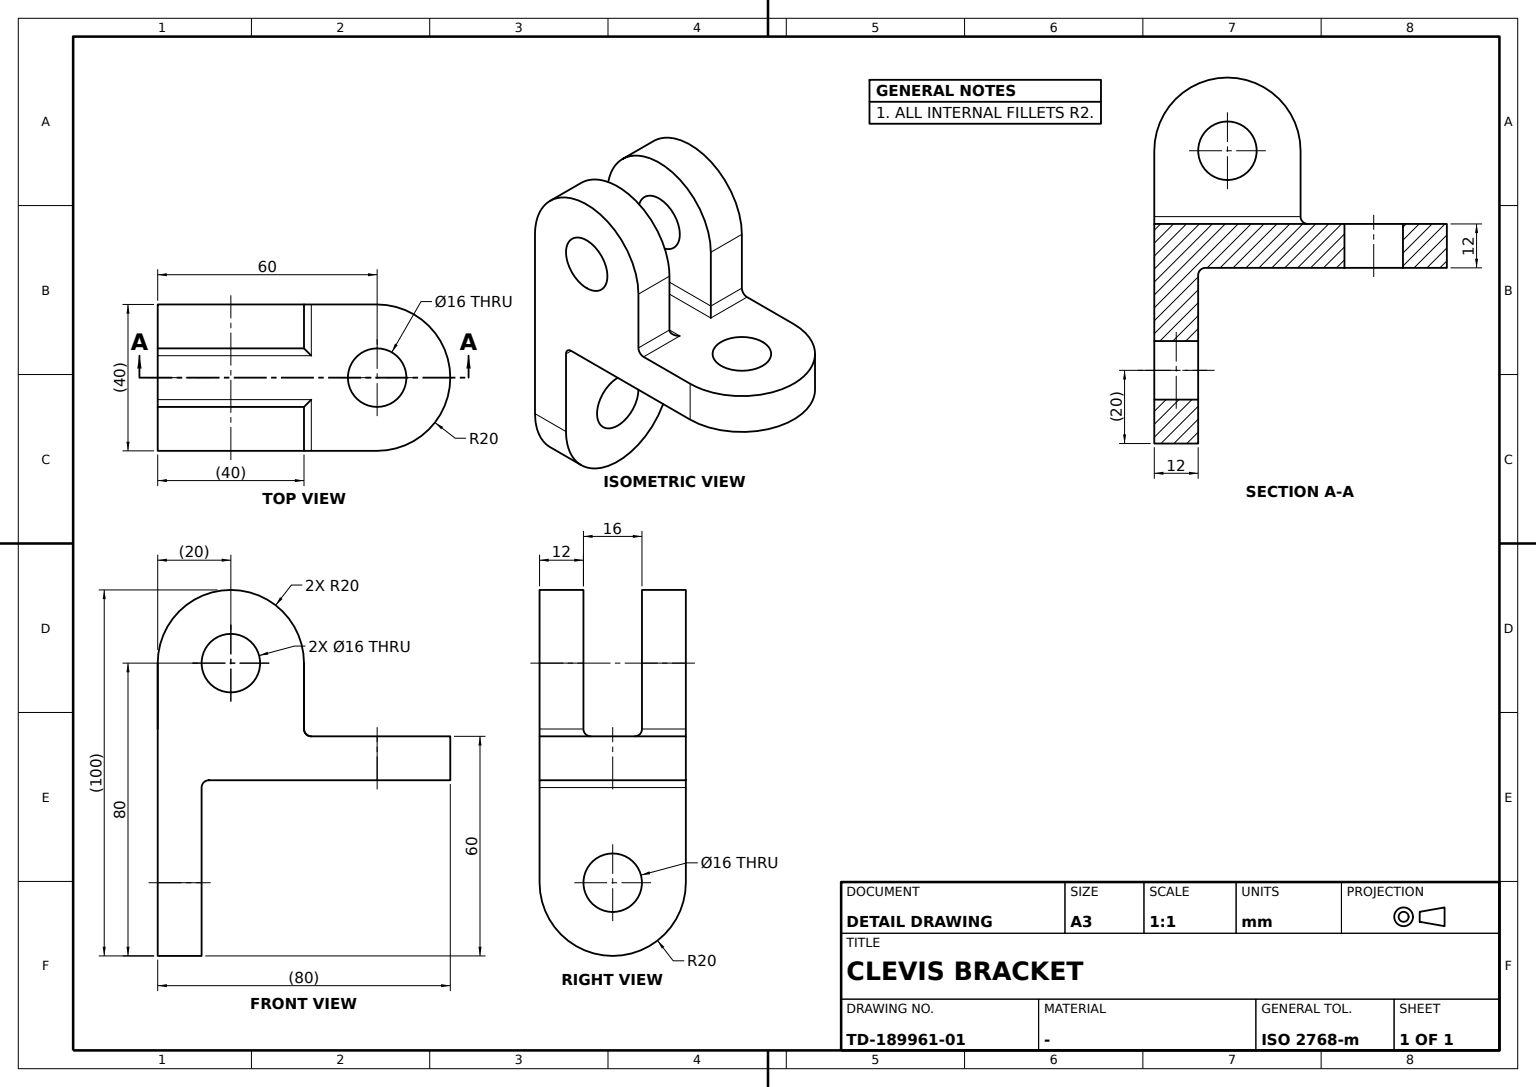
ISO-10303-21;
HEADER;
FILE_DESCRIPTION((''),'2;1');
FILE_NAME('','',(''),(''),'','','');
FILE_SCHEMA(('AUTOMOTIVE_DESIGN'));
ENDSEC;
DATA;
#1=APPLICATION_CONTEXT('');
#2=PRODUCT_CONTEXT('',#1,'mechanical');
#3=PRODUCT('','','',(#2));
#4=PRODUCT_DEFINITION_FORMATION('','',#3);
#5=PRODUCT_DEFINITION_CONTEXT('',#1,'design');
#6=PRODUCT_DEFINITION('','',#4,#5);
#7=PRODUCT_DEFINITION_SHAPE('','',#6);
#8=(LENGTH_UNIT()NAMED_UNIT(*)SI_UNIT(.MILLI.,.METRE.));
#9=(NAMED_UNIT(*)PLANE_ANGLE_UNIT()SI_UNIT($,.RADIAN.));
#10=(NAMED_UNIT(*)SI_UNIT($,.STERADIAN.)SOLID_ANGLE_UNIT());
#11=UNCERTAINTY_MEASURE_WITH_UNIT(LENGTH_MEASURE(0.005),#8,'distance_accuracy_value','');
#12=(GEOMETRIC_REPRESENTATION_CONTEXT(3)GLOBAL_UNCERTAINTY_ASSIGNED_CONTEXT((#11))GLOBAL_UNIT_ASSIGNED_CONTEXT((#8,#9,#10))REPRESENTATION_CONTEXT('',''));
#13=CARTESIAN_POINT('',(-20.,40.,50.));
#14=VERTEX_POINT('',#13);
#15=CARTESIAN_POINT('',(-8.,40.,50.));
#16=VERTEX_POINT('',#15);
#17=CARTESIAN_POINT('',(0.,40.,50.));
#18=DIRECTION('',(1.,0.,0.));
#19=VECTOR('',#18,1000.);
#20=LINE('',#17,#19);
#21=EDGE_CURVE('',#14,#16,#20,.T.);
#22=ORIENTED_EDGE('',*,*,#21,.T.);
#23=CARTESIAN_POINT('',(-8.,40.,32.));
#24=VERTEX_POINT('',#23);
#25=DIRECTION('',(0.,0.,1.));
#26=VECTOR('',#25,1000.);
#27=LINE('',#15,#26);
#28=EDGE_CURVE('',#24,#16,#27,.T.);
#29=ORIENTED_EDGE('',*,*,#28,.F.);
#30=CARTESIAN_POINT('',(-20.,40.,32.));
#31=VERTEX_POINT('',#30);
#32=CARTESIAN_POINT('',(0.,40.,32.));
#33=LINE('',#32,#19);
#34=EDGE_CURVE('',#31,#24,#33,.T.);
#35=ORIENTED_EDGE('',*,*,#34,.F.);
#36=CARTESIAN_POINT('',(-20.,40.,0.));
#37=DIRECTION('',(0.,0.,-1.));
#38=VECTOR('',#37,1000.);
#39=LINE('',#36,#38);
#40=EDGE_CURVE('',#14,#31,#39,.T.);
#41=ORIENTED_EDGE('',*,*,#40,.F.);
#42=EDGE_LOOP('',(#22,#29,#35,#41));
#43=FACE_BOUND('',#42,.T.);
#44=DIRECTION('',(0.,-1.,0.));
#45=AXIS2_PLACEMENT_3D('',#17,#44,#37);
#46=PLANE('',#45);
#47=ADVANCED_FACE('',(#43),#46,.F.);
#48=CARTESIAN_POINT('',(-20.,60.,30.));
#49=VERTEX_POINT('',#48);
#50=CARTESIAN_POINT('',(-20.,60.,18.));
#51=VERTEX_POINT('',#50);
#52=CARTESIAN_POINT('',(-20.,60.,24.));
#53=LINE('',#52,#26);
#54=EDGE_CURVE('',#49,#51,#53,.F.);
#55=ORIENTED_EDGE('',*,*,#54,.F.);
#56=CARTESIAN_POINT('',(20.,60.,30.));
#57=VERTEX_POINT('',#56);
#58=CARTESIAN_POINT('',(0.,60.,30.));
#59=DIRECTION('',(-1.,0.,0.));
#60=AXIS2_PLACEMENT_3D('',#58,#37,#59);
#61=CIRCLE('',#60,20.);
#62=EDGE_CURVE('',#57,#49,#61,.F.);
#63=ORIENTED_EDGE('',*,*,#62,.F.);
#64=CARTESIAN_POINT('',(20.,60.,18.));
#65=VERTEX_POINT('',#64);
#66=CARTESIAN_POINT('',(20.,60.,24.));
#67=LINE('',#66,#26);
#68=EDGE_CURVE('',#57,#65,#67,.F.);
#69=ORIENTED_EDGE('',*,*,#68,.T.);
#70=CARTESIAN_POINT('',(0.,60.,18.));
#71=AXIS2_PLACEMENT_3D('',#70,#25,#18);
#72=CIRCLE('',#71,20.);
#73=EDGE_CURVE('',#65,#51,#72,.T.);
#74=ORIENTED_EDGE('',*,*,#73,.T.);
#75=EDGE_LOOP('',(#55,#63,#69,#74));
#76=FACE_BOUND('',#75,.T.);
#77=CARTESIAN_POINT('',(0.,60.,24.));
#78=AXIS2_PLACEMENT_3D('',#77,#25,#18);
#79=CYLINDRICAL_SURFACE('',#78,20.);
#80=ADVANCED_FACE('',(#76),#79,.T.);
#81=CARTESIAN_POINT('',(0.,0.,-2.));
#82=VERTEX_POINT('',#81);
#83=CARTESIAN_POINT('',(0.,0.,-10.));
#84=DIRECTION('',(0.,1.,0.));
#85=AXIS2_PLACEMENT_3D('',#83,#84,#25);
#86=CIRCLE('',#85,8.);
#87=EDGE_CURVE('',#82,#82,#86,.F.);
#88=ORIENTED_EDGE('',*,*,#87,.F.);
#89=EDGE_LOOP('',(#88));
#90=FACE_BOUND('',#89,.T.);
#91=CARTESIAN_POINT('',(8.,0.,50.));
#92=VERTEX_POINT('',#91);
#93=CARTESIAN_POINT('',(8.,0.,32.));
#94=VERTEX_POINT('',#93);
#95=CARTESIAN_POINT('',(8.,0.,90.));
#96=LINE('',#95,#38);
#97=EDGE_CURVE('',#92,#94,#96,.T.);
#98=ORIENTED_EDGE('',*,*,#97,.T.);
#99=CARTESIAN_POINT('',(6.,0.,30.));
#100=VERTEX_POINT('',#99);
#101=CARTESIAN_POINT('',(6.,0.,32.));
#102=AXIS2_PLACEMENT_3D('',#101,#84,#25);
#103=CIRCLE('',#102,2.);
#104=EDGE_CURVE('',#94,#100,#103,.T.);
#105=ORIENTED_EDGE('',*,*,#104,.T.);
#106=CARTESIAN_POINT('',(-6.,0.,30.));
#107=VERTEX_POINT('',#106);
#108=CARTESIAN_POINT('',(0.,0.,30.));
#109=LINE('',#108,#19);
#110=EDGE_CURVE('',#107,#100,#109,.T.);
#111=ORIENTED_EDGE('',*,*,#110,.F.);
#112=CARTESIAN_POINT('',(-8.,0.,32.));
#113=VERTEX_POINT('',#112);
#114=CARTESIAN_POINT('',(-6.,0.,32.));
#115=AXIS2_PLACEMENT_3D('',#114,#84,#25);
#116=CIRCLE('',#115,2.);
#117=EDGE_CURVE('',#107,#113,#116,.T.);
#118=ORIENTED_EDGE('',*,*,#117,.T.);
#119=CARTESIAN_POINT('',(-8.,0.,50.));
#120=VERTEX_POINT('',#119);
#121=CARTESIAN_POINT('',(-8.,0.,30.));
#122=LINE('',#121,#26);
#123=EDGE_CURVE('',#113,#120,#122,.T.);
#124=ORIENTED_EDGE('',*,*,#123,.T.);
#125=CARTESIAN_POINT('',(-20.,0.,50.));
#126=VERTEX_POINT('',#125);
#127=CARTESIAN_POINT('',(0.,0.,50.));
#128=LINE('',#127,#19);
#129=EDGE_CURVE('',#126,#120,#128,.T.);
#130=ORIENTED_EDGE('',*,*,#129,.F.);
#131=CARTESIAN_POINT('',(-20.,0.,-10.));
#132=VERTEX_POINT('',#131);
#133=CARTESIAN_POINT('',(-20.,0.,0.));
#134=LINE('',#133,#26);
#135=EDGE_CURVE('',#132,#126,#134,.T.);
#136=ORIENTED_EDGE('',*,*,#135,.F.);
#137=CARTESIAN_POINT('',(20.,0.,-10.));
#138=VERTEX_POINT('',#137);
#139=CIRCLE('',#85,20.);
#140=EDGE_CURVE('',#138,#132,#139,.T.);
#141=ORIENTED_EDGE('',*,*,#140,.F.);
#142=CARTESIAN_POINT('',(20.,0.,50.));
#143=VERTEX_POINT('',#142);
#144=CARTESIAN_POINT('',(20.,0.,0.));
#145=LINE('',#144,#26);
#146=EDGE_CURVE('',#138,#143,#145,.T.);
#147=ORIENTED_EDGE('',*,*,#146,.T.);
#148=EDGE_CURVE('',#92,#143,#128,.T.);
#149=ORIENTED_EDGE('',*,*,#148,.F.);
#150=EDGE_LOOP('',(#98,#105,#111,#118,#124,#130,#136,#141,#147,#149));
#151=FACE_BOUND('',#150,.T.);
#152=PLANE('',#85);
#153=ADVANCED_FACE('',(#90,#151),#152,.F.);
#154=CARTESIAN_POINT('',(6.,42.,30.));
#155=VERTEX_POINT('',#154);
#156=CARTESIAN_POINT('',(20.,42.,30.));
#157=VERTEX_POINT('',#156);
#158=CARTESIAN_POINT('',(0.,42.,30.));
#159=LINE('',#158,#19);
#160=EDGE_CURVE('',#155,#157,#159,.T.);
#161=ORIENTED_EDGE('',*,*,#160,.F.);
#162=CARTESIAN_POINT('',(8.,40.,32.));
#163=VERTEX_POINT('',#162);
#164=CARTESIAN_POINT('',(6.,42.,32.));
#165=DIRECTION('',(-0.707106781,-0.707106781,0.));
#166=DIRECTION('',(0.707106781,-0.707106781,0.));
#167=AXIS2_PLACEMENT_3D('',#164,#165,#166);
#168=ELLIPSE('',#167,2.828427,2.);
#169=EDGE_CURVE('',#163,#155,#168,.F.);
#170=ORIENTED_EDGE('',*,*,#169,.F.);
#171=CARTESIAN_POINT('',(20.,40.,32.));
#172=VERTEX_POINT('',#171);
#173=EDGE_CURVE('',#163,#172,#33,.T.);
#174=ORIENTED_EDGE('',*,*,#173,.T.);
#175=CARTESIAN_POINT('',(20.,42.,32.));
#176=AXIS2_PLACEMENT_3D('',#175,#18,#37);
#177=CIRCLE('',#176,2.);
#178=EDGE_CURVE('',#172,#157,#177,.T.);
#179=ORIENTED_EDGE('',*,*,#178,.T.);
#180=EDGE_LOOP('',(#161,#170,#174,#179));
#181=FACE_BOUND('',#180,.T.);
#182=CARTESIAN_POINT('',(0.,42.,32.));
#183=AXIS2_PLACEMENT_3D('',#182,#18,#44);
#184=CYLINDRICAL_SURFACE('',#183,2.);
#185=ADVANCED_FACE('',(#181),#184,.F.);
#186=ORIENTED_EDGE('',*,*,#28,.T.);
#187=CARTESIAN_POINT('',(-8.,20.,50.));
#188=AXIS2_PLACEMENT_3D('',#187,#18,#37);
#189=CIRCLE('',#188,20.);
#190=EDGE_CURVE('',#16,#120,#189,.T.);
#191=ORIENTED_EDGE('',*,*,#190,.T.);
#192=ORIENTED_EDGE('',*,*,#123,.F.);
#193=VECTOR('',#44,1000.);
#194=LINE('',#23,#193);
#195=EDGE_CURVE('',#24,#113,#194,.T.);
#196=ORIENTED_EDGE('',*,*,#195,.F.);
#197=EDGE_LOOP('',(#186,#191,#192,#196));
#198=FACE_BOUND('',#197,.T.);
#199=CARTESIAN_POINT('',(-8.,20.,42.));
#200=VERTEX_POINT('',#199);
#201=CIRCLE('',#188,8.);
#202=EDGE_CURVE('',#200,#200,#201,.T.);
#203=ORIENTED_EDGE('',*,*,#202,.F.);
#204=EDGE_LOOP('',(#203));
#205=FACE_BOUND('',#204,.T.);
#206=CARTESIAN_POINT('',(-8.,40.,30.));
#207=AXIS2_PLACEMENT_3D('',#206,#18,#25);
#208=PLANE('',#207);
#209=ADVANCED_FACE('',(#198,#205),#208,.T.);
#210=CARTESIAN_POINT('',(0.,12.,-18.));
#211=VERTEX_POINT('',#210);
#212=CARTESIAN_POINT('',(0.,12.,-10.));
#213=AXIS2_PLACEMENT_3D('',#212,#44,#37);
#214=CIRCLE('',#213,8.);
#215=EDGE_CURVE('',#211,#211,#214,.T.);
#216=ORIENTED_EDGE('',*,*,#215,.F.);
#217=EDGE_LOOP('',(#216));
#218=FACE_BOUND('',#217,.T.);
#219=ORIENTED_EDGE('',*,*,#87,.T.);
#220=EDGE_LOOP('',(#219));
#221=FACE_BOUND('',#220,.T.);
#222=CARTESIAN_POINT('',(0.,11.9,-10.));
#223=AXIS2_PLACEMENT_3D('',#222,#44,#18);
#224=CYLINDRICAL_SURFACE('',#223,8.);
#225=ADVANCED_FACE('',(#218,#221),#224,.F.);
#226=CARTESIAN_POINT('',(20.,20.,42.));
#227=VERTEX_POINT('',#226);
#228=CARTESIAN_POINT('',(20.,20.,50.));
#229=AXIS2_PLACEMENT_3D('',#228,#18,#37);
#230=CIRCLE('',#229,8.);
#231=EDGE_CURVE('',#227,#227,#230,.T.);
#232=ORIENTED_EDGE('',*,*,#231,.T.);
#233=EDGE_LOOP('',(#232));
#234=FACE_BOUND('',#233,.T.);
#235=CARTESIAN_POINT('',(8.,20.,58.));
#236=VERTEX_POINT('',#235);
#237=CARTESIAN_POINT('',(8.,20.,50.));
#238=AXIS2_PLACEMENT_3D('',#237,#59,#25);
#239=CIRCLE('',#238,8.);
#240=EDGE_CURVE('',#236,#236,#239,.T.);
#241=ORIENTED_EDGE('',*,*,#240,.T.);
#242=EDGE_LOOP('',(#241));
#243=FACE_BOUND('',#242,.T.);
#244=CARTESIAN_POINT('',(19.9,20.,50.));
#245=AXIS2_PLACEMENT_3D('',#244,#59,#84);
#246=CYLINDRICAL_SURFACE('',#245,8.);
#247=ADVANCED_FACE('',(#234,#243),#246,.F.);
#248=CARTESIAN_POINT('',(8.,40.,50.));
#249=VERTEX_POINT('',#248);
#250=CARTESIAN_POINT('',(20.,40.,50.));
#251=VERTEX_POINT('',#250);
#252=EDGE_CURVE('',#249,#251,#20,.T.);
#253=ORIENTED_EDGE('',*,*,#252,.T.);
#254=CARTESIAN_POINT('',(20.,40.,0.));
#255=LINE('',#254,#38);
#256=EDGE_CURVE('',#251,#172,#255,.T.);
#257=ORIENTED_EDGE('',*,*,#256,.T.);
#258=ORIENTED_EDGE('',*,*,#173,.F.);
#259=LINE('',#248,#38);
#260=EDGE_CURVE('',#249,#163,#259,.T.);
#261=ORIENTED_EDGE('',*,*,#260,.F.);
#262=EDGE_LOOP('',(#253,#257,#258,#261));
#263=FACE_BOUND('',#262,.T.);
#264=ADVANCED_FACE('',(#263),#46,.F.);
#265=ORIENTED_EDGE('',*,*,#73,.F.);
#266=CARTESIAN_POINT('',(20.,14.,18.));
#267=VERTEX_POINT('',#266);
#268=CARTESIAN_POINT('',(20.,0.,18.));
#269=LINE('',#268,#193);
#270=EDGE_CURVE('',#65,#267,#269,.T.);
#271=ORIENTED_EDGE('',*,*,#270,.T.);
#272=CARTESIAN_POINT('',(-20.,14.,18.));
#273=VERTEX_POINT('',#272);
#274=CARTESIAN_POINT('',(0.,14.,18.));
#275=LINE('',#274,#19);
#276=EDGE_CURVE('',#273,#267,#275,.T.);
#277=ORIENTED_EDGE('',*,*,#276,.F.);
#278=CARTESIAN_POINT('',(-20.,0.,18.));
#279=LINE('',#278,#193);
#280=EDGE_CURVE('',#51,#273,#279,.T.);
#281=ORIENTED_EDGE('',*,*,#280,.F.);
#282=EDGE_LOOP('',(#265,#271,#277,#281));
#283=FACE_BOUND('',#282,.T.);
#284=CARTESIAN_POINT('',(8.,60.,18.));
#285=VERTEX_POINT('',#284);
#286=CIRCLE('',#71,8.);
#287=EDGE_CURVE('',#285,#285,#286,.T.);
#288=ORIENTED_EDGE('',*,*,#287,.T.);
#289=EDGE_LOOP('',(#288));
#290=FACE_BOUND('',#289,.T.);
#291=AXIS2_PLACEMENT_3D('',#70,#25,#44);
#292=PLANE('',#291);
#293=ADVANCED_FACE('',(#283,#290),#292,.F.);
#294=ORIENTED_EDGE('',*,*,#202,.T.);
#295=EDGE_LOOP('',(#294));
#296=FACE_BOUND('',#295,.T.);
#297=CARTESIAN_POINT('',(-20.,20.,42.));
#298=VERTEX_POINT('',#297);
#299=CARTESIAN_POINT('',(-20.,20.,50.));
#300=AXIS2_PLACEMENT_3D('',#299,#18,#37);
#301=CIRCLE('',#300,8.);
#302=EDGE_CURVE('',#298,#298,#301,.F.);
#303=ORIENTED_EDGE('',*,*,#302,.T.);
#304=EDGE_LOOP('',(#303));
#305=FACE_BOUND('',#304,.T.);
#306=ADVANCED_FACE('',(#296,#305),#246,.F.);
#307=ORIENTED_EDGE('',*,*,#215,.T.);
#308=EDGE_LOOP('',(#307));
#309=FACE_BOUND('',#308,.T.);
#310=CARTESIAN_POINT('',(20.,12.,16.));
#311=VERTEX_POINT('',#310);
#312=CARTESIAN_POINT('',(20.,12.,-10.));
#313=VERTEX_POINT('',#312);
#314=CARTESIAN_POINT('',(20.,12.,0.));
#315=LINE('',#314,#38);
#316=EDGE_CURVE('',#311,#313,#315,.T.);
#317=ORIENTED_EDGE('',*,*,#316,.T.);
#318=CARTESIAN_POINT('',(-20.,12.,-10.));
#319=VERTEX_POINT('',#318);
#320=CIRCLE('',#213,20.);
#321=EDGE_CURVE('',#313,#319,#320,.F.);
#322=ORIENTED_EDGE('',*,*,#321,.T.);
#323=CARTESIAN_POINT('',(-20.,12.,16.));
#324=VERTEX_POINT('',#323);
#325=CARTESIAN_POINT('',(-20.,12.,0.));
#326=LINE('',#325,#38);
#327=EDGE_CURVE('',#324,#319,#326,.T.);
#328=ORIENTED_EDGE('',*,*,#327,.F.);
#329=CARTESIAN_POINT('',(0.,12.,16.));
#330=LINE('',#329,#19);
#331=EDGE_CURVE('',#324,#311,#330,.T.);
#332=ORIENTED_EDGE('',*,*,#331,.T.);
#333=EDGE_LOOP('',(#317,#322,#328,#332));
#334=FACE_BOUND('',#333,.T.);
#335=CARTESIAN_POINT('',(0.,12.,18.));
#336=AXIS2_PLACEMENT_3D('',#335,#44,#37);
#337=PLANE('',#336);
#338=ADVANCED_FACE('',(#309,#334),#337,.F.);
#339=ORIENTED_EDGE('',*,*,#21,.F.);
#340=CIRCLE('',#300,20.);
#341=EDGE_CURVE('',#14,#126,#340,.T.);
#342=ORIENTED_EDGE('',*,*,#341,.T.);
#343=ORIENTED_EDGE('',*,*,#129,.T.);
#344=ORIENTED_EDGE('',*,*,#190,.F.);
#345=EDGE_LOOP('',(#339,#342,#343,#344));
#346=FACE_BOUND('',#345,.T.);
#347=CARTESIAN_POINT('',(0.,20.,50.));
#348=AXIS2_PLACEMENT_3D('',#347,#18,#84);
#349=CYLINDRICAL_SURFACE('',#348,20.);
#350=ADVANCED_FACE('',(#346),#349,.T.);
#351=CARTESIAN_POINT('',(-6.,42.,30.));
#352=VERTEX_POINT('',#351);
#353=CARTESIAN_POINT('',(-6.,40.,30.));
#354=LINE('',#353,#193);
#355=EDGE_CURVE('',#352,#107,#354,.T.);
#356=ORIENTED_EDGE('',*,*,#355,.F.);
#357=CARTESIAN_POINT('',(-6.,42.,32.));
#358=DIRECTION('',(0.707106781,0.707106781,0.));
#359=AXIS2_PLACEMENT_3D('',#357,#166,#358);
#360=ELLIPSE('',#359,2.828427,2.);
#361=EDGE_CURVE('',#24,#352,#360,.T.);
#362=ORIENTED_EDGE('',*,*,#361,.F.);
#363=ORIENTED_EDGE('',*,*,#195,.T.);
#364=ORIENTED_EDGE('',*,*,#117,.F.);
#365=EDGE_LOOP('',(#356,#362,#363,#364));
#366=FACE_BOUND('',#365,.T.);
#367=CARTESIAN_POINT('',(-6.,40.,32.));
#368=AXIS2_PLACEMENT_3D('',#367,#44,#59);
#369=CYLINDRICAL_SURFACE('',#368,2.);
#370=ADVANCED_FACE('',(#366),#369,.F.);
#371=ORIENTED_EDGE('',*,*,#140,.T.);
#372=CARTESIAN_POINT('',(-20.,6.,-10.));
#373=VECTOR('',#84,1000.);
#374=LINE('',#372,#373);
#375=EDGE_CURVE('',#319,#132,#374,.F.);
#376=ORIENTED_EDGE('',*,*,#375,.F.);
#377=ORIENTED_EDGE('',*,*,#321,.F.);
#378=CARTESIAN_POINT('',(20.,6.,-10.));
#379=LINE('',#378,#373);
#380=EDGE_CURVE('',#313,#138,#379,.F.);
#381=ORIENTED_EDGE('',*,*,#380,.T.);
#382=EDGE_LOOP('',(#371,#376,#377,#381));
#383=FACE_BOUND('',#382,.T.);
#384=CARTESIAN_POINT('',(0.,6.,-10.));
#385=AXIS2_PLACEMENT_3D('',#384,#84,#59);
#386=CYLINDRICAL_SURFACE('',#385,20.);
#387=ADVANCED_FACE('',(#383),#386,.T.);
#388=LINE('',#162,#193);
#389=EDGE_CURVE('',#163,#94,#388,.T.);
#390=ORIENTED_EDGE('',*,*,#389,.F.);
#391=ORIENTED_EDGE('',*,*,#169,.T.);
#392=CARTESIAN_POINT('',(6.,40.,30.));
#393=LINE('',#392,#193);
#394=EDGE_CURVE('',#155,#100,#393,.T.);
#395=ORIENTED_EDGE('',*,*,#394,.T.);
#396=ORIENTED_EDGE('',*,*,#104,.F.);
#397=EDGE_LOOP('',(#390,#391,#395,#396));
#398=FACE_BOUND('',#397,.T.);
#399=CARTESIAN_POINT('',(6.,40.,32.));
#400=AXIS2_PLACEMENT_3D('',#399,#44,#18);
#401=CYLINDRICAL_SURFACE('',#400,2.);
#402=ADVANCED_FACE('',(#398),#401,.F.);
#403=CARTESIAN_POINT('',(-20.,42.,30.));
#404=VERTEX_POINT('',#403);
#405=CARTESIAN_POINT('',(-20.,42.,32.));
#406=AXIS2_PLACEMENT_3D('',#405,#18,#37);
#407=CIRCLE('',#406,2.);
#408=EDGE_CURVE('',#31,#404,#407,.T.);
#409=ORIENTED_EDGE('',*,*,#408,.F.);
#410=ORIENTED_EDGE('',*,*,#34,.T.);
#411=ORIENTED_EDGE('',*,*,#361,.T.);
#412=EDGE_CURVE('',#404,#352,#159,.T.);
#413=ORIENTED_EDGE('',*,*,#412,.F.);
#414=EDGE_LOOP('',(#409,#410,#411,#413));
#415=FACE_BOUND('',#414,.T.);
#416=ADVANCED_FACE('',(#415),#184,.F.);
#417=ORIENTED_EDGE('',*,*,#252,.F.);
#418=CIRCLE('',#238,20.);
#419=EDGE_CURVE('',#92,#249,#418,.T.);
#420=ORIENTED_EDGE('',*,*,#419,.F.);
#421=ORIENTED_EDGE('',*,*,#148,.T.);
#422=CIRCLE('',#229,20.);
#423=EDGE_CURVE('',#251,#143,#422,.T.);
#424=ORIENTED_EDGE('',*,*,#423,.F.);
#425=EDGE_LOOP('',(#417,#420,#421,#424));
#426=FACE_BOUND('',#425,.T.);
#427=ADVANCED_FACE('',(#426),#349,.T.);
#428=CARTESIAN_POINT('',(-20.,14.,16.));
#429=AXIS2_PLACEMENT_3D('',#428,#18,#37);
#430=CIRCLE('',#429,2.);
#431=EDGE_CURVE('',#273,#324,#430,.T.);
#432=ORIENTED_EDGE('',*,*,#431,.F.);
#433=ORIENTED_EDGE('',*,*,#276,.T.);
#434=CARTESIAN_POINT('',(20.,14.,16.));
#435=AXIS2_PLACEMENT_3D('',#434,#18,#37);
#436=CIRCLE('',#435,2.);
#437=EDGE_CURVE('',#267,#311,#436,.T.);
#438=ORIENTED_EDGE('',*,*,#437,.T.);
#439=ORIENTED_EDGE('',*,*,#331,.F.);
#440=EDGE_LOOP('',(#432,#433,#438,#439));
#441=FACE_BOUND('',#440,.T.);
#442=CARTESIAN_POINT('',(0.,14.,16.));
#443=AXIS2_PLACEMENT_3D('',#442,#18,#25);
#444=CYLINDRICAL_SURFACE('',#443,2.);
#445=ADVANCED_FACE('',(#441),#444,.F.);
#446=ORIENTED_EDGE('',*,*,#97,.F.);
#447=ORIENTED_EDGE('',*,*,#419,.T.);
#448=ORIENTED_EDGE('',*,*,#260,.T.);
#449=ORIENTED_EDGE('',*,*,#389,.T.);
#450=EDGE_LOOP('',(#446,#447,#448,#449));
#451=FACE_BOUND('',#450,.T.);
#452=ORIENTED_EDGE('',*,*,#240,.F.);
#453=EDGE_LOOP('',(#452));
#454=FACE_BOUND('',#453,.T.);
#455=CARTESIAN_POINT('',(8.,40.,90.));
#456=AXIS2_PLACEMENT_3D('',#455,#59,#37);
#457=PLANE('',#456);
#458=ADVANCED_FACE('',(#451,#454),#457,.T.);
#459=ORIENTED_EDGE('',*,*,#280,.T.);
#460=ORIENTED_EDGE('',*,*,#431,.T.);
#461=ORIENTED_EDGE('',*,*,#327,.T.);
#462=ORIENTED_EDGE('',*,*,#375,.T.);
#463=ORIENTED_EDGE('',*,*,#135,.T.);
#464=ORIENTED_EDGE('',*,*,#341,.F.);
#465=ORIENTED_EDGE('',*,*,#40,.T.);
#466=ORIENTED_EDGE('',*,*,#408,.T.);
#467=CARTESIAN_POINT('',(-20.,0.,30.));
#468=LINE('',#467,#373);
#469=EDGE_CURVE('',#404,#49,#468,.T.);
#470=ORIENTED_EDGE('',*,*,#469,.T.);
#471=ORIENTED_EDGE('',*,*,#54,.T.);
#472=EDGE_LOOP('',(#459,#460,#461,#462,#463,#464,#465,#466,#470,#471));
#473=FACE_BOUND('',#472,.T.);
#474=ORIENTED_EDGE('',*,*,#302,.F.);
#475=EDGE_LOOP('',(#474));
#476=FACE_BOUND('',#475,.T.);
#477=AXIS2_PLACEMENT_3D('',#133,#18,#84);
#478=PLANE('',#477);
#479=ADVANCED_FACE('',(#473,#476),#478,.F.);
#480=ORIENTED_EDGE('',*,*,#62,.T.);
#481=ORIENTED_EDGE('',*,*,#469,.F.);
#482=ORIENTED_EDGE('',*,*,#412,.T.);
#483=ORIENTED_EDGE('',*,*,#355,.T.);
#484=ORIENTED_EDGE('',*,*,#110,.T.);
#485=ORIENTED_EDGE('',*,*,#394,.F.);
#486=ORIENTED_EDGE('',*,*,#160,.T.);
#487=CARTESIAN_POINT('',(20.,0.,30.));
#488=LINE('',#487,#373);
#489=EDGE_CURVE('',#157,#57,#488,.T.);
#490=ORIENTED_EDGE('',*,*,#489,.T.);
#491=EDGE_LOOP('',(#480,#481,#482,#483,#484,#485,#486,#490));
#492=FACE_BOUND('',#491,.T.);
#493=CARTESIAN_POINT('',(-8.,60.,30.));
#494=VERTEX_POINT('',#493);
#495=CIRCLE('',#60,8.);
#496=EDGE_CURVE('',#494,#494,#495,.T.);
#497=ORIENTED_EDGE('',*,*,#496,.T.);
#498=EDGE_LOOP('',(#497));
#499=FACE_BOUND('',#498,.T.);
#500=CARTESIAN_POINT('',(0.,40.,30.));
#501=AXIS2_PLACEMENT_3D('',#500,#37,#84);
#502=PLANE('',#501);
#503=ADVANCED_FACE('',(#492,#499),#502,.F.);
#504=ORIENTED_EDGE('',*,*,#496,.F.);
#505=EDGE_LOOP('',(#504));
#506=FACE_BOUND('',#505,.T.);
#507=ORIENTED_EDGE('',*,*,#287,.F.);
#508=EDGE_LOOP('',(#507));
#509=FACE_BOUND('',#508,.T.);
#510=CARTESIAN_POINT('',(0.,60.,29.9));
#511=AXIS2_PLACEMENT_3D('',#510,#37,#18);
#512=CYLINDRICAL_SURFACE('',#511,8.);
#513=ADVANCED_FACE('',(#506,#509),#512,.F.);
#514=ORIENTED_EDGE('',*,*,#231,.F.);
#515=EDGE_LOOP('',(#514));
#516=FACE_BOUND('',#515,.T.);
#517=ORIENTED_EDGE('',*,*,#270,.F.);
#518=ORIENTED_EDGE('',*,*,#68,.F.);
#519=ORIENTED_EDGE('',*,*,#489,.F.);
#520=ORIENTED_EDGE('',*,*,#178,.F.);
#521=ORIENTED_EDGE('',*,*,#256,.F.);
#522=ORIENTED_EDGE('',*,*,#423,.T.);
#523=ORIENTED_EDGE('',*,*,#146,.F.);
#524=ORIENTED_EDGE('',*,*,#380,.F.);
#525=ORIENTED_EDGE('',*,*,#316,.F.);
#526=ORIENTED_EDGE('',*,*,#437,.F.);
#527=EDGE_LOOP('',(#517,#518,#519,#520,#521,#522,#523,#524,#525,#526));
#528=FACE_BOUND('',#527,.T.);
#529=AXIS2_PLACEMENT_3D('',#144,#18,#84);
#530=PLANE('',#529);
#531=ADVANCED_FACE('',(#516,#528),#530,.T.);
#532=CLOSED_SHELL('',(#47,#80,#153,#185,#209,#225,#247,#264,#293,#306,#338,#350,#370,#387,#402,#416,#427,#445,#458,#479,#503,#513,#531));
#533=MANIFOLD_SOLID_BREP('',#532);
#534=ADVANCED_BREP_SHAPE_REPRESENTATION('',(#533),#12);
#535=SHAPE_DEFINITION_REPRESENTATION(#7,#534);
ENDSEC;
END-ISO-10303-21;
